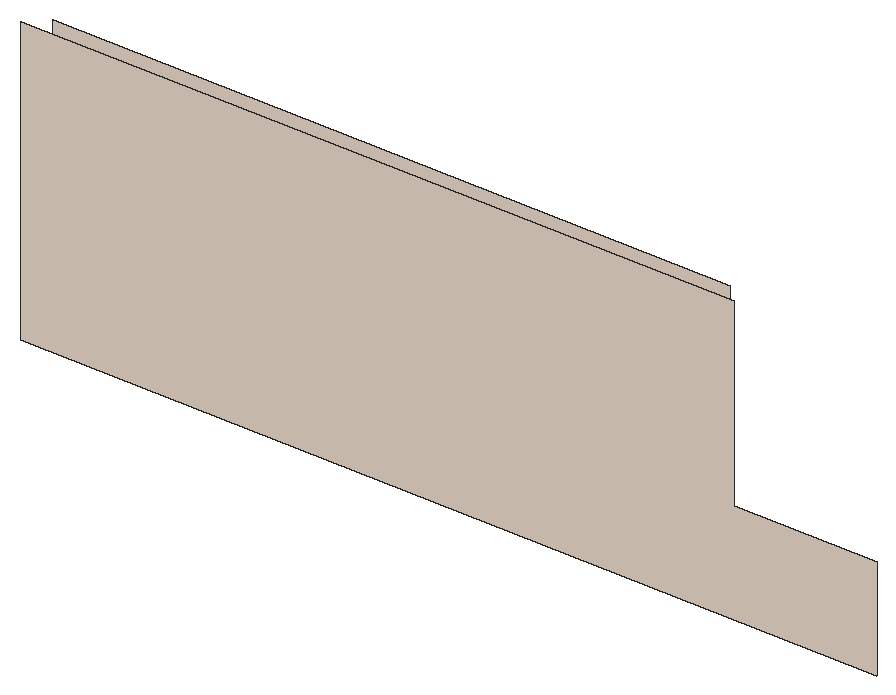
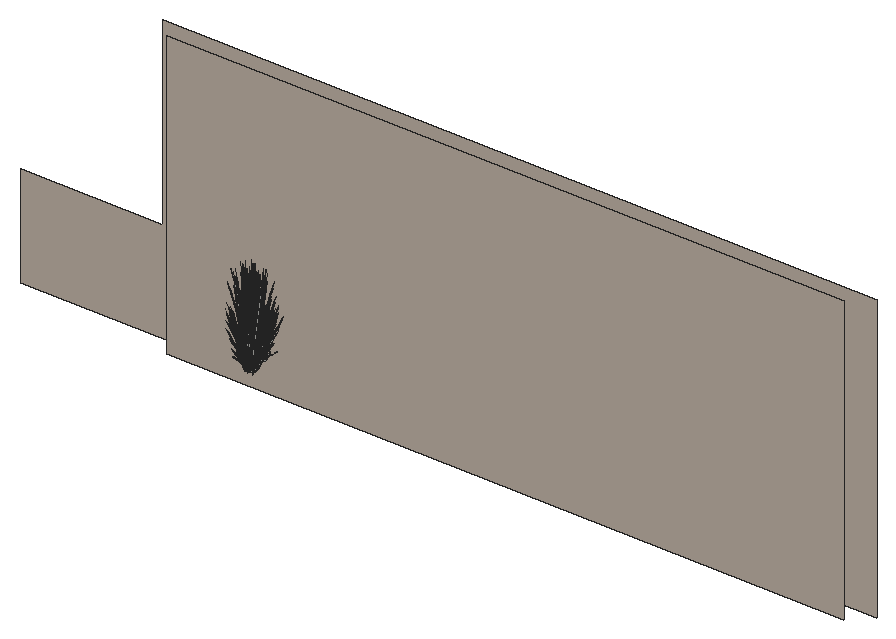
# SketchUp Ruby script. Lengths in inches.
U = 1.inch
M = Sketchup.active_model
def pt(a) = Geom::Point3d.new(a.map { |v| v * U })
def face(e, loops, mat)
  f = e.add_face(loops[0].map { |a| pt(a) })
  loops[1..].each { |l| e.add_face(l.map { |a| pt(a) }).erase! }
  f.material = f.back_material = mat if mat
  f
end
# faces: each face lists its corners as indices into pts; further lists are holes
def faces(e, pts, list, mat = nil) = list.each { |f| face(e, (f[0].is_a?(Array) ? f : [f]).map { |l| l.map { |i| pts[i] } }, mat) }
# xy, xz, yz: faces in a plane at the given z, y or x. An outline is a flat list of corners, or four numbers for a rectangle; further outlines are holes
def ring(l) = l.size == 4 ? [[l[0], l[1]], [l[2], l[1]], [l[2], l[3]], [l[0], l[3]]] : l.each_slice(2).to_a
def flat(e, list, mat, &to3) = list.each { |f| face(e, (f[0].is_a?(Array) ? f : [f]).map { |l| ring(l).map { |u, v| to3.(u, v) } }, mat) }
def xy(e, z, list, mat = nil) = flat(e, list, mat) { |x, y| [x, y, z] }
def xz(e, y, list, mat = nil) = flat(e, list, mat) { |x, z| [x, y, z] }
def yz(e, x, list, mat = nil) = flat(e, list, mat) { |y, z| [x, y, z] }
def lines(e, pts, list) = list.each { |a, b| e.add_line(pt(pts[a]), pt(pts[b])) }
# prism: a flat outline (further loops are holes) pulled along v
def prism(e, loops, v, mat = nil)
  f = face(e, loops, mat); d = Geom::Vector3d.new(v.map { |x| x * U })
  f.pushpull(f.normal.samedirection?(d) ? d.length : -d.length)
end
def box(e, o, s, mat = nil) = prism(e, [[o, [o[0] + s[0], o[1], o[2]], [o[0] + s[0], o[1] + s[1], o[2]], [o[0], o[1] + s[1], o[2]]]], [0, 0, s[2]], mat)
def at(x, y, z, deg = 0) = Geom::Transformation.translation(pt([x, y, z])) * Geom::Transformation.rotation(ORIGIN, Z_AXIS, deg.degrees)
def axes(o, x, y, z) = Geom::Transformation.new([*x, 0, *y, 0, *z, 0, *pt(o).to_a, 1])
def part(name) = M.definitions.add(name)
# library, detail: a bought-in or finely detailed component or shape, given as its bounding box
def library(name, o, s) = part(name).tap { |d| box(d.entities, o, s) }
def detail(e, o, s) = box(e.add_group.entities, o, s)
def put(e, d, t, mat = nil) = e.add_instance(d, t).tap { |i| i.material = mat if mat }
def group(e, t, mat = nil) = e.add_group.tap { |g| g.transformation = t; g.material = mat if mat }.entities
root = M.entities
M.materials.add("C01_Vanilla_Cream").color = [244, 228, 212]
M.materials.add("LightPink_Translucent").color = [144, 107, 117]
M.materials["LightPink_Translucent"].alpha = 0.75
c1 = part("blade")
p = [[2.15,0.21,22],[0,0.17,0],[0.09,0.45,0],[2.18,0.31,22],[2.29,0.31,22],[0.38,0.45,0],
  [2.48,0.24,33],[2.49,0.24,33],[2.48,0.22,33]]
faces(c1.entities,p,[[0,1,2,3],[4,5,2,3],[6,3,4,7],[8,0,3,6]])
c2 = part("seeds")
p = [[0.3,-0.1,1.38],[-0.01,-0.03,1.59],[-0.01,-0.03,0.03],[0.14,-0.07,-0.07],[0.29,-0.03,3],[0.15,0.01,3.11]]
faces(c2.entities,p,[[0,1,2,3],[1,0,4,5]],"LightPink_Translucent")
c3 = part("blade with seeds")
put(c3.entities,c1,at(0,0,0))
put(c3.entities,c2,axes([2.4,0.25,30.99],[1.5799,-0.05474,1.17369],[-0.12525,1.92788,0.29478],[-0.07173,-0.02425,1.56792]))
xz(root,0,[[0,0,432,0,432,51.56,360,51.56,360,144,0,144]],"C01_Vanilla_Cream")
xz(root,9,[[9,0,351,144]],"C01_Vanilla_Cream")
put(root,c3,axes([294.87,22.27,19.51],[0.23093,-0.01116,1.28532],[-0.15319,0.4836,0.10393],[-0.32909,-0.02991,0.54946]))
put(root,c3,axes([294.97,23.12,19.51],[0.19317,-0.10421,1.28532],[0.16263,0.48153,0.10393],[-0.30326,0.10883,0.54946]))
put(root,c3,axes([294.37,23.9375,18.55],[0.19348,0.04044,1.07251],[0.1247,0.41309,-0.23066],[-0.26282,0.07733,0.45856]))
put(root,c3,axes([296.08,22.62,19.11],[0.15825,-0.07127,1.32798],[0.05457,0.4976,0.10393],[-0.34278,0.06603,0.47463]))
put(root,c3,axes([294.375,22.95,20.14],[-0.09091,0.06396,1.31208],[0.00773,0.46734,-0.2075],[-0.20839,0.06078,0.10523]))
put(root,c3,axes([295.5625,21.82,20.34],[-0.55654,-0.01186,-0.53284],[0.03738,-0.49951,0.0643],[-0.23578,-0.05271,0.75375]))
put(root,c3,axes([295.11,21.94,18.55],[0.1087,0.13716,1.07251],[-0.25048,0.37284,-0.23066],[-0.25719,-0.08912,0.45856]))
put(root,c3,axes([294.67,22.68,20],[-0.46269,-0.13744,-0.2656],[0.13495,-0.40096,0.3429],[-0.18628,0.03677,0.65611]))
put(root,c3,axes([295.31,21.49,19.51],[0.2068,0.08488,1.28532],[-0.42797,0.35609,0.10393],[-0.26673,-0.16064,0.54946]))
put(root,c3,axes([293.37,23.42,20.13],[0.07105,0.01321,1.33037],[0.2198,0.43529,-0.12571],[-0.14545,0.11425,0.23543]))
put(root,c3,axes([294.99,22.89,20.11],[-0.15083,0.44814,-0.38324],[-0.51712,-0.15361,-0.29685],[-0.2082,0.04109,0.7333]))
put(root,c3,axes([295.38,21.92,20.11],[-0.40426,0.32635,-0.38324],[-0.35404,-0.34474,-0.29685],[-0.2054,-0.04965,0.7333]))
put(root,c3,axes([294.73,22.86,17.72],[0.01412,0.07764,1.32257],[-0.28464,0.40547,-0.20205],[-0.20218,-0.02044,0.22528]))
put(root,c3,axes([294.81,21,20.13],[0.04127,0.04917,1.33037],[-0.19898,0.44196,-0.12571],[-0.20151,0.0032,0.23543]))
put(root,c3,axes([293.96,24.8,18.68],[0.23202,-0.22328,0.86145],[0.09155,0.35348,0.63294],[-0.16768,0.06329,0.18974]))
put(root,c3,axes([295.27,20.71,20.14],[-0.11979,-0.00348,1.31208],[-0.38137,0.34775,-0.2075],[-0.20349,-0.07106,0.10523]))
put(root,c3,axes([294.78,22.63,20.15],[0.15729,-0.44921,0.36002],[0.51712,0.15361,0.29685],[-0.20336,0.027,0.74497]))
put(root,c3,axes([294.96,22.5,20.38],[0.28012,0.44611,-0.0912],[-0.49717,0.21923,-0.50621],[-0.20951,0.05886,0.76918]))
put(root,c3,axes([295.59,21.58,20.38],[-0.02981,0.50103,-0.0912],[-0.56442,-0.01369,-0.50621],[-0.21738,-0.0348,0.76918]))
put(root,c3,axes([295.23,21.61,20],[-0.31678,-0.30846,-0.2656],[0.36171,-0.29199,0.3429],[-0.18378,-0.04443,0.65611]))
put(root,c3,axes([294.74,22.51,20.15],[-0.20448,-0.33592,0.04823],[0.37288,-0.16442,0.37966],[-0.16437,0.03244,0.57892]))
put(root,c3,axes([295.67,23.44,19.51],[0.13906,-0.15138,1.28532],[0.35111,0.40859,0.10393],[-0.24082,0.18608,0.54946]))
put(root,c3,axes([294.84,23.84,20],[-0.48462,0.07041,-0.2656],[-0.12797,-0.4025,0.3429],[-0.13888,0.10811,0.65611]))
put(root,c3,axes([294.57,25.03,17.72],[0.07468,0.04922,1.32257],[0.12663,0.45605,-0.20205],[-0.16551,0.09725,0.22528]))
put(root,c3,axes([294.47,22.35,18.68],[0.35544,-0.03525,0.86145],[-0.22547,0.31061,0.63294],[-0.17565,-0.04659,0.18974]))
put(root,c3,axes([294.9,23.75,20.15],[-0.13808,-0.45342,0.36002],[0.54163,-0.07869,0.29685],[-0.15963,0.10664,0.74497]))
put(root,c3,axes([295.18,21.5,20.42],[0.45978,-0.36358,0.40322],[0.39653,0.38611,0.33247],[-0.21571,-0.06707,0.83437]))
put(root,c3,axes([294.79,23.66,20.15],[-0.3822,-0.20719,0.04823],[0.22252,-0.29505,0.37966],[-0.12254,0.09539,0.57892]))
put(root,c3,axes([295.57,23.82,19.51],[0.10366,-0.16934,1.28532],[0.43488,0.35044,0.10393],[-0.19618,0.21841,0.54946]))
put(root,c3,axes([295.16,22.64,20.39],[0.46269,0.13744,0.2656],[-0.13495,0.40096,-0.3429],[-0.18628,0.03677,0.65611]))
put(root,c3,axes([295.24,23.89,20.11],[0.14302,0.44985,-0.38324],[-0.54163,0.07869,-0.29685],[-0.15522,0.12083,0.7333]))
put(root,c3,axes([295.39,21.49,20.15],[0.02803,-0.37463,0.04823],[0.42332,0.01027,0.37966],[-0.16216,-0.0392,0.57892]))
put(root,c3,axes([294.39,24.69,20.14],[-0.01384,0.09749,1.31208],[0.39274,0.33916,-0.2075],[-0.10282,0.16039,0.10523]))
put(root,c3,axes([296.59,23.5625,18.15],[-0.57914,-0.08077,-0.46765],[0.12221,-0.49823,-0.12274],[-0.17283,-0.06037,1.03225]))
put(root,c3,axes([296.69,20.85,20.67],[-0.37157,0.4723,-0.10215],[-0.5381,-0.2721,-0.56695],[-0.18705,-0.13344,0.86148]))
put(root,c3,axes([295.68,21.77,20.39],[0.31678,0.30846,0.2656],[-0.36171,0.29199,-0.3429],[-0.18378,-0.04443,0.65611]))
put(root,c3,axes([296.53,21.23,20.34],[-0.47473,-0.23813,-0.53284],[0.33738,-0.41728,0.0643],[-0.172,-0.14218,0.75375]))
put(root,c3,axes([296.31,21.24,20.11],[-0.54938,0.11711,-0.38324],[-0.0961,-0.44351,-0.29685],[-0.14756,-0.1271,0.7333]))
put(root,c3,axes([295.83,24.51,18.12],[-0.52105,-0.24633,-0.37238],[0.31144,-0.44171,0],[-0.11867,-0.0561,1.18128]))
put(root,c3,axes([295.6,20.84,17.72],[-0.05393,0.0649,1.32257],[-0.545,0.13993,-0.20205],[-0.13166,-0.12729,0.22528]))
put(root,c3,axes([294.98,23.5625,20.38],[0.515,0.27165,-0.0912],[-0.2967,0.3934,-0.50621],[-0.1455,0.13675,0.76918]))
put(root,c3,axes([296.15,24.8,18.38],[-0.34808,0.49367,0],[-0.58235,-0.27531,-0.38706],[-0.13264,-0.0627,1.22783]))
put(root,c3,axes([294.13,24.74,20.84],[0.49129,0.13151,-0.04866],[-0.15113,0.40475,-0.22062],[-0.08035,0.06145,0.72768]))
put(root,c3,axes([295.23,23.6,20.39],[0.48462,-0.07041,0.2656],[0.12797,0.4025,-0.3429],[-0.13888,0.10811,0.65611]))
put(root,c3,axes([295.51,25.52,18.55],[0.17569,-0.07772,1.07251],[0.43377,0.23434,-0.23066],[-0.12911,0.20277,0.45856]))
put(root,c3,axes([295.26,21.09,18.2],[-0.1606,0.40228,-0.02919],[-0.4943,-0.12375,-0.13237],[-0.07505,-0.0658,0.43661]))
put(root,c3,axes([296.55,19.72,20.13],[-0.01039,0.05905,1.33037],[-0.51226,0.21431,-0.12571],[-0.15074,-0.10955,0.23543]))
put(root,c3,axes([296,20.58,18.55],[-0.03371,0.16116,1.07251],[-0.49286,0.13491,-0.23066],[-0.11521,-0.20831,0.45856]))
put(root,c3,axes([296.16,21,19.51],[0.12726,0.15818,1.28532],[-0.58807,0.13317,0.10393],[-0.13291,-0.24832,0.54946]))
put(root,c3,axes([297.25,23.64,18.6],[-0.56211,0.32708,-0.21822],[-0.3738,-0.46216,-0.37502],[-0.13869,-0.04694,1.19781]))
put(root,c3,axes([295.69,24.67,20.15],[-0.39645,-0.33614,0.36002],[0.42102,-0.2899,0.29685],[-0.07313,0.15771,0.74497]))
put(root,c3,axes([296.37,20.91,20],[-0.08599,-0.39682,-0.2656],[0.49155,-0.10478,0.3429],[-0.13203,-0.11372,0.65611]))
put(root,c3,axes([295,22.92,18.38],[-0.69617,0,0],[0,-0.55062,-0.38706],[0,-0.12541,1.22783]))
put(root,c3,axes([295.97,24.32,18.125],[-0.13078,-0.42928,-0.23233],[0.51941,-0.1219,0.23233],[-0.10471,-0.0495,1.0423]))
put(root,c3,axes([295.55,24.64,20.15],[-0.45752,-0.02296,0.04823],[0.01254,-0.34663,0.37966],[-0.04787,0.13278,0.57892]))
put(root,c3,axes([295.69,24.77,20],[-0.3767,0.25939,-0.2656],[-0.3566,-0.29618,0.3429],[-0.05426,0.15048,0.65611]))
put(root,c3,axes([297.62,23.99,18.15],[-0.375,0.3703,-0.46765],[-0.46584,-0.33578,-0.12274],[-0.15027,0.09237,1.03225]))
put(root,c3,axes([296.66,21.24,20.39],[0.08599,0.39682,0.2656],[-0.49155,0.10478,-0.3429],[-0.13203,-0.11372,0.65611]))
put(root,c3,axes([294.35,25.69,20.13],[0.06316,-0.02974,1.33037],[0.52204,0.19785,-0.12571],[-0.01227,0.16473,0.23543]))
put(root,c3,axes([295.53,22.78,18.35],[-0.51786,0.4142,0.23067],[-0.51817,-0.40984,-0.27369],[-0.01808,-0.11762,1.23664]))
put(root,c3,axes([297.67,23.92,19.1],[0.48111,0.19866,1.13446],[-0.47133,0.42798,0.44862],[-0.21112,-0.25366,0.95105]))
put(root,c3,axes([295.83,20.32,18.68],[0.29042,0.17147,0.86145],[-0.42295,0.10307,0.63294],[-0.0905,-0.13178,0.18974]))
put(root,c3,axes([297.875,23.79,18.45],[-0.54364,-0.39653,-0.18894],[0.45745,-0.44527,0.41347],[-0.14639,0.04639,1.26162]))
put(root,c3,axes([296.89,23.4,18.26],[-0.33445,-0.41351,-0.33554],[0.50659,-0.29119,0.16149],[-0.10823,-0.05117,1.07733]))
put(root,c3,axes([295.94,24.5,20.61],[-0.01449,0.45571,-0.59145],[-0.61002,-0.03061,0.07138],[-0.06438,0.19306,0.83667]))
put(root,c3,axes([295.93,25.78,18.68],[-0.01441,-0.29294,0.86145],[0.36003,0.20894,0.63294],[-0.07081,0.13963,0.18974]))
put(root,c3,axes([296.4375,20.77,20.42],[0.62019,-0.12663,0.40322],[0.10763,0.49673,0.33247],[-0.14586,-0.1464,0.83437]))
put(root,c3,axes([297.6,23.7,18.26],[-0.60457,0.03041,-0.33554],[-0.05467,-0.50484,0.16149],[-0.10823,0.05117,1.07733]))
put(root,c3,axes([296.58,20.88,20.15],[0.25304,-0.31296,0.04823],[0.36033,0.18221,0.37966],[-0.11649,-0.10034,0.57892]))
put(root,c3,axes([296.45,24.55,18.46],[0.52105,0.24633,0.37238],[-0.31144,0.44171,0],[-0.11867,-0.0561,1.18128]))
put(root,c3,axes([295.74,25.14,19.125],[0.01223,-0.25433,1.15759],[0.55017,0.13434,0.15997],[-0.04767,0.27105,0.54661]))
put(root,c3,axes([296.9375,23.64,18.43],[0.14756,-0.58378,-0.17572],[0.69966,0.10176,0.38453],[-0.12225,-0.08062,1.1733]))
put(root,c3,axes([297.19,23.78,18.5625],[-0.1074,0.43968,0.1086],[-0.52474,-0.07632,-0.3101],[-0.0955,-0.04515,0.95058]))
put(root,c3,axes([297.13,19.95,20.14],[-0.08515,-0.06907,1.31208],[-0.56828,0.04379,-0.2075],[-0.0907,-0.16522,0.10523]))
put(root,c3,axes([298.24,25,18.12],[-0.52105,0.24633,-0.37238],[-0.31144,-0.44171,0],[-0.11867,0.0561,1.18128]))
put(root,c3,axes([295.15,22.55,18.12],[0,-0.49266,-0.37238],[0.62289,0,0],[0,-0.11221,1.18128]))
put(root,c3,axes([295.42,23.01,18.46],[0,0.49266,0.37238],[-0.62289,0,0],[0,-0.11221,1.18128]))
put(root,c3,axes([298.27,24.87,18.25],[-0.34375,-0.4954,-0.03857],[0.58235,-0.27531,0.38706],[-0.1435,0.04717,1.22723]))
put(root,c3,axes([296.07,24.65,20.36],[0.39855,0.33102,-0.4254],[-0.42102,0.2899,-0.32951],[-0.06064,0.16819,0.81396]))
put(root,c3,axes([298.11,24.81,18.125],[-0.51941,-0.1219,-0.23233],[0.13078,-0.42928,0.23233],[-0.10471,0.0495,1.0423]))
put(root,c3,axes([295.89,24.4,20.39],[0.3767,-0.25939,0.2656],[0.3566,0.29618,-0.3429],[-0.05426,0.15048,0.65611]))
put(root,c3,axes([296.78,23.12,18.6],[-0.62699,-0.23507,-0.21822],[0.3019,-0.49615,-0.37502],[-0.0197,-0.12182,1.19781]))
put(root,c3,axes([298.41,22.97,18.73],[-0.01521,-0.46386,1.05954],[0.68831,0.12024,0.44862],[-0.1628,0.25382,1.00012]))
put(root,c3,axes([295.65,24.47,20.65],[0.61188,0.02441,-0.10123],[-0.01672,0.46217,-0.56189],[-0.0425,0.178,0.85379]))
put(root,c3,axes([295.63,25.15,18.72],[0.50577,-0.08724,0.04881],[0.11627,0.35148,-0.64728],[-0.03206,0.17792,0.5802]))
put(root,c3,axes([298.02,23.57,18.6],[0.06488,0.56215,-0.21822],[-0.6757,0.03399,-0.37502],[-0.11898,0.07488,1.19781]))
put(root,c3,axes([296.5,22.62,18.18],[-0.22864,-0.5052,-0.52377],[0.65862,-0.18195,-0.13747],[-0.02527,-0.17107,1.15612]))
put(root,c3,axes([298,21.02,20.38],[-0.54481,0.22937,-0.0912],[-0.26773,-0.4071,-0.50621],[-0.07188,-0.17155,0.76918]))
put(root,c3,axes([297.53,21.04,20.11],[-0.54728,-0.1235,-0.38324],[0.18759,-0.42344,-0.29685],[-0.05018,-0.17048,0.7333]))
put(root,c3,axes([296.52,24.17,19.51],[-0.01363,-0.18909,1.28532],[0.5906,0.12544,0.10393],[-0.03653,0.26947,0.54946]))
put(root,c3,axes([295.42,22.5625,18.125],[0.38863,-0.30738,-0.23233],[0.38863,0.30738,0.23233],[0,-0.09901,1.0423]))
put(root,c3,axes([297.17,20.57,18.2],[-0.38473,0.28263,-0.02919],[-0.35252,-0.30954,-0.13237],[-0.02482,-0.08771,0.43661]))
put(root,c3,axes([297.02,23.36,18.37],[0.70367,0.1038,0.34316],[-0.1432,0.58624,0.13466],[-0.10283,-0.05661,1.19142]))
put(root,c3,axes([296.84,23.25,18.64],[-0.27012,0.44393,0.33554],[-0.56127,-0.21365,-0.16149],[0,-0.10233,1.07733]))
put(root,c3,axes([297.73,21.12,20.34],[-0.26572,-0.40059,-0.53284],[0.54698,-0.22325,0.0643],[-0.06214,-0.19355,0.75375]))
put(root,c3,axes([296.64,24.3,18.46],[0.59825,-0.13076,0.13232],[0.14773,0.48663,0.26315],[-0.05336,-0.0709,1.20305]))
put(root,c3,axes([297.41,24.375,18.25],[-0.56127,-0.22118,0],[0.27012,-0.45959,0],[0,0,1.2203]))
put(root,c3,axes([297.83,21.17,20.39],[-0.16784,0.37886,0.2656],[-0.48968,-0.1105,-0.3429],[-0.0449,-0.15254,0.65611]))
put(root,c3,axes([298.71,24.93,18.38],[0.34808,0.49367,0],[-0.58235,0.27531,-0.38706],[-0.13264,0.0627,1.22783]))
put(root,c3,axes([296.9375,25.14,20.4],[-0.54859,-0.1288,0.39962],[0.18759,-0.42344,0.32951],[0.03297,0.16652,0.82692]))
put(root,c3,axes([296.79,25.17,20.15],[-0.41024,0.16744,0.04823],[-0.2008,-0.30532,0.37966],[0.03962,0.13459,0.57892]))
put(root,c3,axes([298.42,24.32,18.46],[0.16083,-0.48962,0.13232],[0.58854,0.13856,0.26315],[-0.10167,0.00238,1.20305]))
put(root,c3,axes([298.15,23.67,18.5625],[0.41131,0.296,0.1086],[-0.34309,0.33395,-0.3101],[-0.0955,0.04515,0.95058]))
put(root,c3,axes([298,23.31,18.33],[-0.51786,-0.42404,-0.04598],[0.51817,-0.4243,0],[-0.01808,-0.01481,1.31678]))
put(root,c3,axes([298.14,23.46,18.64],[0.60457,-0.03041,0.33554],[0.05467,0.50484,-0.16149],[-0.10823,0.05117,1.07733]))
put(root,c3,axes([298.29,24.62,18.35],[0.697,0.16013,0.23067],[-0.17437,0.57237,-0.27369],[-0.11536,0.07164,1.23664]))
put(root,c3,axes([297.27,20.23,17.72],[-0.09338,0.01775,1.32257],[-0.51641,-0.1998,-0.20205],[0.00867,-0.16666,0.22528]))
put(root,c3,axes([298.59,24.59,18.46],[0.52105,-0.24633,0.37238],[0.31144,0.44171,0],[-0.11867,0.0561,1.18128]))
put(root,c3,axes([297.78,20.78,20],[0.16784,-0.37886,-0.2656],[0.48968,0.1105,0.3429],[-0.0449,-0.15254,0.65611]))
put(root,c3,axes([296.96,22.82,18.37],[0.24206,0.5509,0.34316],[-0.69162,0.19157,0.13466],[0.00845,-0.10123,1.19142]))
put(root,c3,axes([296.85,22.75,18.26],[0.27012,-0.44393,-0.33554],[0.56127,0.21365,0.16149],[0,-0.10233,1.07733]))
put(root,c3,axes([297.54,24.18,18.26],[-0.18165,-0.42474,0],[0.51872,-0.14874,0],[0,0,1.15778]))
put(root,c3,axes([296.88,25.08,17.72],[0.0901,-0.02681,1.32257],[0.54199,0.14755,-0.20205],[0.01585,0.1663,0.22528]))
put(root,c3,axes([297,25.23,20],[-0.16784,0.37886,-0.2656],[-0.48968,-0.1105,0.3429],[0.0449,0.15254,0.65611]))
put(root,c3,axes([298.27,23.35,18.26],[-0.27012,0.44393,-0.33554],[-0.56127,-0.21365,0.16149],[0,0.10233,1.07733]))
put(root,c3,axes([297.98,20.83,20.15],[0.41024,-0.16744,0.04823],[0.2008,0.30532,0.37966],[-0.03962,-0.13459,0.57892]))
put(root,c3,axes([296.65,25.9,20.14],[0.07057,0.07933,1.31208],[0.56952,0.03117,-0.2075],[0.05727,0.17496,0.10523]))
put(root,c3,axes([299.34,23.07,18.46],[-0.43742,-0.35886,0.13232],[0.44081,-0.34807,0.26315],[-0.04831,0.07329,1.20305]))
put(root,c3,axes([297.83,22.87,18.26],[0,-0.57005,0],[0.69617,0,0],[0,0,1.34592]))
put(root,c3,axes([297.84,20.86,20.15],[0.54859,0.1288,0.36002],[-0.18759,0.42344,0.29685],[-0.03297,-0.16652,0.74497]))
put(root,c3,axes([297.18,22.97,18.43],[0.6273,0.23878,0.18048],[-0.3019,0.49615,0.37502],[0,-0.11437,1.20407]))
put(root,c3,axes([298.18,23.1,18.32],[0,0.56976,-0.04228],[-0.69617,0,0],[0,0.01791,1.34526]))
put(root,c3,axes([296.98,22.64,18.64],[-0.60457,0.03041,0.33554],[-0.05467,-0.50484,-0.16149],[0.10823,-0.05117,1.07733]))
put(root,c3,axes([296.94,24.83,20.39],[0.16784,-0.37886,0.2656],[0.48968,0.1105,-0.3429],[0.0449,0.15254,0.65611]))
put(root,c3,axes([296.7,21.77,18.46],[-0.16083,0.48962,0.13232],[-0.58854,-0.13856,0.26315],[0.10167,-0.00238,1.20305]))
put(root,c3,axes([297.85,24.2,18.32],[0.24206,0.56598,-0.04509],[-0.69162,0.19832,0],[0.00845,0.01976,1.2913]))
put(root,c3,axes([296.41,21.17,18.38],[-0.34808,-0.49367,0],[0.58235,-0.27531,-0.38706],[0.13264,-0.0627,1.22783]))
put(root,c3,axes([297.05,24.89,20.34],[0.26572,0.40059,-0.53284],[-0.54698,0.22325,0.0643],[0.06214,0.19355,0.75375]))
put(root,c3,axes([299.84,23.46,18.25],[-0.69582,-0.00394,-0.03732],[0,-0.55062,0.37457],[-0.02187,0.12535,1.18764]))
put(root,c3,axes([298.48,21.8,18.46],[-0.59825,0.13076,0.13232],[-0.14773,-0.48663,0.26315],[0.05336,0.0709,1.20305]))
put(root,c3,axes([297.87,19.98,18.68],[0.07142,0.28728,0.86145],[-0.3962,-0.15911,0.63294],[0.04263,-0.1471,0.18974]))
put(root,c3,axes([297.6,26.18,20.84],[0.38473,-0.28263,-0.04866],[0.35252,0.30954,-0.22062],[0.02482,0.08771,0.72768]))
put(root,c3,axes([297.5,22.51,18.37],[-0.46162,0.4471,0.34316],[-0.54842,-0.39467,0.13466],[0.11129,-0.04462,1.19142]))
put(root,c3,axes([298.29,23.21,18.26],[0.38863,0.31822,0],[-0.38863,0.31822,0],[0,0,1.2695]))
put(root,c3,axes([298.28,22.84,18.64],[0.27012,-0.44393,0.33554],[0.56127,0.21365,-0.16149],[0,0.10233,1.07733]))
put(root,c3,axes([298.05,24.38,18.26],[0.56127,0.22118,0],[-0.27012,0.45959,0],[0,0,1.31215]))
put(root,c3,axes([297.25,24.97,20.11],[0.54728,0.1235,-0.38324],[-0.18759,0.42344,-0.29685],[0.05018,0.17048,0.7333]))
put(root,c3,axes([296.78,24.99,20.38],[0.54481,-0.22937,-0.0912],[0.26773,0.4071,-0.50621],[0.07188,0.17155,0.76918]))
put(root,c3,axes([298.1,22.74,18.39],[-0.70367,-0.1038,0.36899],[0.1432,-0.58624,0.1448],[0.10283,0.05661,1.2811]))
put(root,c3,axes([299.5625,20.44,20.13],[-0.05654,0.03763,1.33037],[-0.55396,-0.12696,-0.12571],[-0.02005,-0.16422,0.23543]))
put(root,c3,axes([299.13,21.53,20.38],[-0.61188,-0.02441,-0.0912],[0.01672,-0.46217,-0.50621],[0.0425,-0.178,0.76918]))
put(root,c3,axes([299.7,23.54,18.125],[-0.38863,0.30738,-0.23233],[-0.38863,-0.30738,0.23233],[0,0.09901,1.0423]))
put(root,c3,axes([298.59,23.48,18.17],[0.20414,0.45107,-0.51909],[-0.58805,0.16245,-0.13624],[0.02256,0.15274,1.1458]))
put(root,c3,axes([298.3,23,18.26],[0.62289,0,0],[0,0.51004,0],[0,0,1.33805]))
put(root,c3,axes([298.89,21.6,20.39],[-0.3767,0.25939,0.2656],[-0.3566,-0.29618,-0.3429],[0.05426,-0.15048,0.65611]))
put(root,c3,axes([297.7,22.43,18.64],[-0.33445,-0.41351,0.33554],[0.50659,-0.29119,-0.16149],[0.10823,0.05117,1.07733]))
put(root,c3,axes([297.09,22.53,18.6],[-0.06488,-0.56215,-0.21822],[0.6757,-0.03399,-0.37502],[0.11898,-0.07488,1.19781]))
put(root,c3,axes([298.52,22.94,18.5625],[0.51872,-0.14368,0.1086],[0.18165,0.41027,-0.3101],[0,0.09029,0.95058]))
put(root,c3,axes([298.71,21.36,20.11],[-0.39855,-0.33102,-0.38324],[0.42102,-0.2899,-0.29685],[0.06064,-0.16819,0.7333]))
put(root,c3,axes([298.34,22.98,18.6],[0.62699,0.23507,-0.21822],[-0.3019,0.49615,-0.37502],[0.0197,0.12182,1.19781]))
put(root,c3,axes([297,21.29,18.125],[0.51941,0.1219,-0.23233],[-0.13078,0.42928,0.23233],[0.10471,-0.0495,1.0423]))
put(root,c3,axes([298.45,20.77,18.55],[-0.15825,0.09972,1.07251],[-0.47395,-0.17454,-0.23066],[0.08785,-0.21706,0.45856]))
put(root,c3,axes([299.7,23.09,18.46],[0,-0.49266,0.37238],[0.62289,0,0],[0,0.11221,1.18128]))
put(root,c3,axes([299.97,23.55,18.12],[0,0.49266,-0.37238],[-0.62289,0,0],[0,0.11221,1.18128]))
put(root,c3,axes([298.3,25.04,20.15],[-0.55374,0.11306,0.36002],[-0.0961,-0.44351,0.29685],[0.13023,0.13071,0.74497]))
put(root,c3,axes([296.88,21.09,18.12],[0.52105,-0.24633,-0.37238],[0.31144,0.44171,0],[0.11867,-0.0561,1.18128]))
put(root,c3,axes([298.2,25.125,20.15],[-0.25304,0.31296,0.04823],[-0.36033,-0.18221,0.37966],[0.11649,0.10034,0.57892]))
put(root,c3,axes([297.56,24.1,19.51],[-0.12726,-0.15818,1.28532],[0.58807,-0.13317,0.10393],[0.13291,0.24832,0.54946]))
put(root,c3,axes([297.93,22.32,18.5625],[0.1074,-0.43968,0.1086],[0.52474,0.07632,-0.3101],[0.0955,0.04515,0.95058]))
put(root,c3,axes([298.67,21.55,18.46],[-0.52105,-0.24633,0.37238],[0.31144,-0.44171,0],[0.11867,0.0561,1.18128]))
put(root,c3,axes([298.83,21.51,20.34],[0.01449,-0.45571,-0.53284],[0.61002,0.03061,0.0643],[0.06438,-0.19306,0.75375]))
put(root,c3,axes([298.22,24.125,18.24],[0.5845,-0.16716,-0.14398],[0.20539,0.48152,0.00006],[0.06452,-0.01848,1.30423]))
put(root,c3,axes([298.12,24.77,20.39],[-0.08599,-0.39682,0.2656],[0.49155,-0.10478,-0.3429],[0.13203,0.11372,0.65611]))
put(root,c3,axes([298.23,22.69,18.26],[0.33445,0.41351,-0.33554],[-0.50659,0.29119,0.16149],[0.10823,0.05117,1.07733]))
put(root,c3,axes([298.45,22.48,19.96],[-0.48108,-0.25598,1.03712],[0.50798,-0.39855,0.44749],[0.15521,0.24018,1.00248]))
put(root,c3,axes([299.09,21.23,20],[0.3767,-0.25939,-0.2656],[0.3566,0.29618,0.3429],[0.05426,-0.15048,0.65611]))
put(root,c3,axes([297.64,25.32,20.13],[0.00165,-0.05965,1.33037],[0.47711,-0.26315,-0.12571],[0.16572,0.09393,0.23543]))
put(root,c3,axes([299.23,21.37,20.15],[0.45752,0.02296,0.04823],[-0.01254,0.34663,0.37966],[0.04787,-0.13278,0.57892]))
put(root,c3,axes([299.18,24.57,18.68],[-0.31347,-0.14166,0.86145],[0.40476,-0.14393,0.63294],[0.10917,0.12192,0.18974]))
put(root,c3,axes([298.06,24.42,18.55],[0.00982,-0.16331,1.07251],[0.4695,-0.18242,-0.23066],[0.14493,0.19547,0.45856]))
put(root,c3,axes([299.68,20.8,20.14],[-0.00537,-0.09805,1.31208],[-0.45391,-0.28338,-0.2075],[0.07018,-0.17178,0.10523]))
put(root,c3,axes([297.5,22.1,18.15],[0.375,-0.3703,-0.46765],[0.46584,0.33578,-0.12274],[0.15027,-0.09237,1.03225]))
put(root,c3,axes([299.08,21.33,20.15],[0.39645,0.33614,0.36002],[-0.42102,0.2899,0.29685],[0.07313,-0.15771,0.74497]))
put(root,c3,axes([299.14,21.77,18.125],[0.13078,0.42928,-0.23233],[-0.51941,0.1219,0.23233],[0.10471,0.0495,1.0423]))
put(root,c3,axes([300.12,23.17,18.38],[0.69617,0,0],[0,0.55062,-0.38706],[0,0.12541,1.22783]))
put(root,c3,axes([297.87,22.46,18.6],[0.56211,-0.32708,-0.21822],[0.3738,0.46216,-0.37502],[0.13869,0.04694,1.19781]))
put(root,c3,axes([299.23,25.21,18.6],[-0.35702,-0.01545,0.78795],[0.23577,-0.32816,0.43504],[0.14104,0.11659,0.61808]))
put(root,c3,axes([299.54,22.4,20.39],[-0.48462,0.07041,0.2656],[-0.12797,-0.4025,-0.3429],[0.13888,-0.10811,0.65611]))
put(root,c3,axes([298.15,21.28,19.51],[-0.10366,0.16934,1.28532],[-0.43488,-0.35044,0.10393],[0.19618,-0.21841,0.54946]))
put(root,c3,axes([298.07,24.97,20.38],[0.33176,-0.4217,-0.0912],[0.48044,0.24295,-0.50621],[0.16701,0.11914,0.76918]))
put(root,c3,axes([296.45,22.17,17.8],[-0.548,0.19724,0.96696],[-0.17442,-0.56594,0.37572],[0.3365,0.00941,1.09981]))
put(root,c3,axes([299.79,22.44,20.38],[-0.515,-0.27165,-0.0912],[0.2967,-0.3934,-0.50621],[0.1455,-0.13675,0.76918]))
put(root,c3,axes([298.47,24.76,20.11],[0.54938,-0.11711,-0.38324],[0.0961,0.44351,-0.29685],[0.14756,0.1271,0.7333]))
